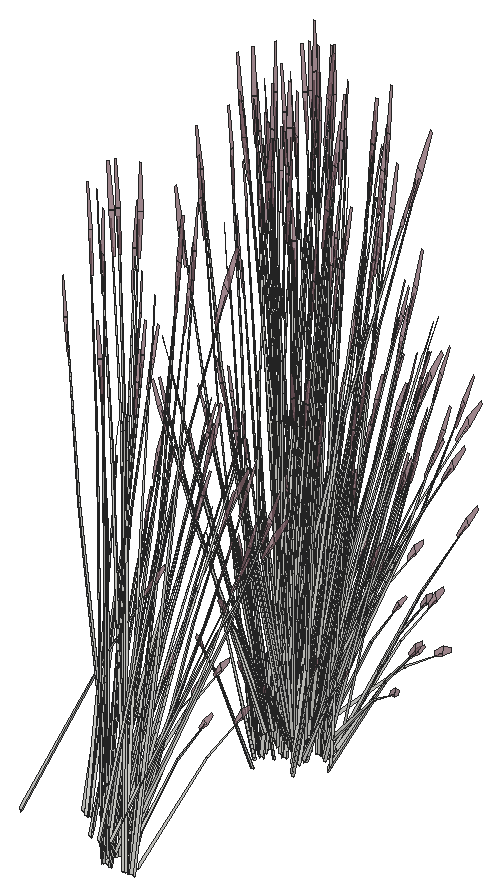
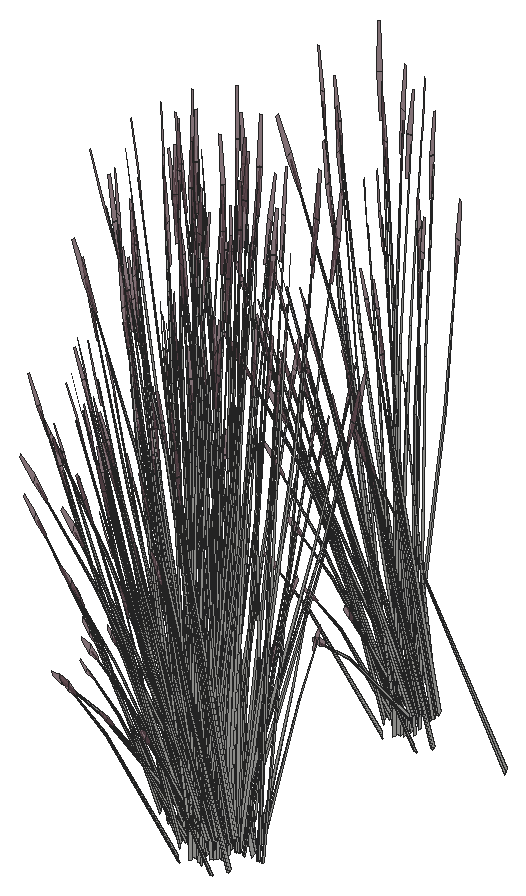
# SketchUp Ruby script. Lengths in inches.
U = 1.inch
M = Sketchup.active_model
def pt(a) = Geom::Point3d.new(a.map { |v| v * U })
def face(e, loops, mat)
  f = e.add_face(loops[0].map { |a| pt(a) })
  loops[1..].each { |l| e.add_face(l.map { |a| pt(a) }).erase! }
  f.material = f.back_material = mat if mat
  f
end
# faces: each face lists its corners as indices into pts; further lists are holes
def faces(e, pts, list, mat = nil) = list.each { |f| face(e, (f[0].is_a?(Array) ? f : [f]).map { |l| l.map { |i| pts[i] } }, mat) }
# xy, xz, yz: faces in a plane at the given z, y or x. An outline is a flat list of corners, or four numbers for a rectangle; further outlines are holes
def ring(l) = l.size == 4 ? [[l[0], l[1]], [l[2], l[1]], [l[2], l[3]], [l[0], l[3]]] : l.each_slice(2).to_a
def flat(e, list, mat, &to3) = list.each { |f| face(e, (f[0].is_a?(Array) ? f : [f]).map { |l| ring(l).map { |u, v| to3.(u, v) } }, mat) }
def xy(e, z, list, mat = nil) = flat(e, list, mat) { |x, y| [x, y, z] }
def xz(e, y, list, mat = nil) = flat(e, list, mat) { |x, z| [x, y, z] }
def yz(e, x, list, mat = nil) = flat(e, list, mat) { |y, z| [x, y, z] }
def lines(e, pts, list) = list.each { |a, b| e.add_line(pt(pts[a]), pt(pts[b])) }
# prism: a flat outline (further loops are holes) pulled along v
def prism(e, loops, v, mat = nil)
  f = face(e, loops, mat); d = Geom::Vector3d.new(v.map { |x| x * U })
  f.pushpull(f.normal.samedirection?(d) ? d.length : -d.length)
end
def box(e, o, s, mat = nil) = prism(e, [[o, [o[0] + s[0], o[1], o[2]], [o[0] + s[0], o[1] + s[1], o[2]], [o[0], o[1] + s[1], o[2]]]], [0, 0, s[2]], mat)
def at(x, y, z, deg = 0) = Geom::Transformation.translation(pt([x, y, z])) * Geom::Transformation.rotation(ORIGIN, Z_AXIS, deg.degrees)
def axes(o, x, y, z) = Geom::Transformation.new([*x, 0, *y, 0, *z, 0, *pt(o).to_a, 1])
def part(name) = M.definitions.add(name)
# library, detail: a bought-in or finely detailed component or shape, given as its bounding box
def library(name, o, s) = part(name).tap { |d| box(d.entities, o, s) }
def detail(e, o, s) = box(e.add_group.entities, o, s)
def put(e, d, t, mat = nil) = e.add_instance(d, t).tap { |i| i.material = mat if mat }
def group(e, t, mat = nil) = e.add_group.tap { |g| g.transformation = t; g.material = mat if mat }.entities
root = M.entities
M.materials.add("LightPink_Translucent").color = [144, 107, 117]
M.materials["LightPink_Translucent"].alpha = 0.75
c1 = part("blade")
p = [[2.15,0.21,22],[0,0.17,0],[0.09,0.45,0],[2.18,0.31,22],[2.29,0.31,22],[0.38,0.45,0],
  [2.48,0.24,33],[2.49,0.24,33],[2.48,0.22,33]]
faces(c1.entities,p,[[0,1,2,3],[4,5,2,3],[6,3,4,7],[8,0,3,6]])
c2 = part("seeds")
p = [[0.3,-0.1,1.38],[-0.01,-0.03,1.59],[-0.01,-0.03,0.03],[0.14,-0.07,-0.07],[0.29,-0.03,3],[0.15,0.01,3.11]]
faces(c2.entities,p,[[0,1,2,3],[1,0,4,5]],"LightPink_Translucent")
c3 = part("blade with seeds")
put(c3.entities,c1,at(0,0,0))
put(c3.entities,c2,axes([2.4,0.25,30.99],[1.5799,-0.05474,1.17369],[-0.12525,1.92788,0.29478],[-0.07173,-0.02425,1.56792]))
put(root,c3,axes([507.35,187.09,1.81],[0.56134,0.36712,0.1448],[-0.46823,0.41419,-0.41347],[-0.13033,0.05599,1.26744]))
put(root,c3,axes([508.8,187.72,4.17],[0.75952,0.01471,-0.71045],[-0.05101,0.61953,0.08574],[0.32177,0.06538,1.00501]))
put(root,c3,axes([507.94,188.22,1.67],[0.7111,-0.30552,0.49651],[0.42504,0.54784,0],[-0.16196,0.06958,1.57504]))
put(root,c3,axes([506.93,187.74,1.48],[0.33034,0.70197,-0.06012],[-0.94388,0.24598,0],[0.01154,0.02451,1.72173]))
put(root,c3,axes([507.3,188.5,1.22],[-0.70886,-0.15119,-0.30978],[0.17848,-0.53243,0.30978],[-0.1429,0.0614,1.38974]))
put(root,c3,axes([510.04,186.47,1.57],[0.95008,0,0],[0,0.68292,-0.51607],[0,0.15554,1.63711]))
put(root,c3,axes([509.66,186.82,1.39],[-0.94962,-0.00489,-0.04976],[0,-0.68292,0.49943],[-0.02984,0.15546,1.58352]))
put(root,c3,axes([507.6,186.22,1.86],[0.85568,0.29155,-0.29095],[-0.41201,0.61537,-0.50002],[0.02689,0.15109,1.59708]))
put(root,c3,axes([509.26,187.98,3.72],[0.43232,0.38257,-0.35414],[-0.49364,0.36215,0.4572],[0.25081,0.0551,0.87481]))
put(root,c3,axes([509.46,186.92,1.22],[-0.53038,0.38124,-0.30978],[-0.53038,-0.38124,0.30978],[0,0.1228,1.38974]))
put(root,c3,axes([507.18,186.95,1.86],[0.08854,0.69723,-0.29095],[-0.92215,0.04216,-0.50002],[-0.16238,0.09287,1.59708]))
put(root,c3,axes([509.03,188.125,3.92],[-0.03826,0.46465,0.0643],[-0.57772,-0.01274,0.50621],[0.2213,0.04862,0.77189]))
put(root,c3,axes([507.51,186.68,1.4],[-0.36864,0.55059,-0.44739],[-0.76598,-0.26498,0.21531],[0,0.12692,1.43643]))
put(root,c3,axes([497.26,188.9,1.78],[-0.18299,-0.15028,1.43002],[0.23809,-0.49714,-0.30754],[0.37023,0.06735,0.61141]))
put(root,c3,axes([509.09,187.98,3.93],[-0.56024,0.40262,0.48003],[-0.48318,-0.42758,0.3958],[0.26285,0.07427,0.9933]))
put(root,c3,axes([507.31,188.44,4.24],[-0.11735,-0.49217,0.35414],[0.67083,-0.12996,-0.4572],[0.18018,0.14104,0.87481]))
put(root,c3,axes([507.53,188.26,1.52],[0.95122,0.19861,0.30756],[-0.23797,0.7099,-0.36492],[-0.15744,0.08885,1.64885]))
put(root,c3,axes([509.83,186.93,1.21],[0,0.61104,-0.49651],[-0.85008,0,0],[0,0.13917,1.57504]))
put(root,c3,axes([507.7,187,3.07],[-0.28223,-0.10528,1.71376],[0.58406,-0.44165,0.13857],[0.36402,0.19924,0.73262]))
put(root,c3,axes([507.76,185.61,3.67],[-0.65655,-0.31748,1.38283],[0.69326,-0.49431,0.59665],[0.21183,0.29789,1.33663]))
put(root,c3,axes([508.75,188.2,1.96],[-0.4278,-0.1757,1.1486],[0.5524,-0.17852,0.84392],[0.14899,0.15122,0.25299]))
put(root,c3,axes([507.24,188.7,4.23],[0.45276,-0.52302,-0.1216],[0.65568,0.30132,-0.67495],[0.22792,0.14777,1.02557]))
put(root,c3,axes([504.26,187.99,4.24],[0.5141,-0.32171,0.35414],[0.48666,0.36734,-0.4572],[-0.07405,0.18664,0.87481]))
put(root,c3,axes([508.11,188.64,1.57],[0.47504,0.61229,0],[-0.79476,0.34146,-0.51607],[-0.18101,0.07777,1.63711]))
put(root,c3,axes([506.65,189.13,3.9],[0.00225,-0.07398,1.77383],[0.65113,-0.32638,-0.16761],[0.22617,0.1165,0.31391]))
put(root,c3,axes([508.87,188.85,0.6875],[0.05536,-0.08822,1.76342],[0.69692,-0.25981,-0.26939],[0.21129,0.13447,0.30037]))
put(root,c3,axes([507.71,186.22,2.03],[-0.02076,-0.57531,1.41272],[0.93937,0.14913,0.59816],[-0.22217,0.31481,1.3335]))
put(root,c3,axes([507.95,186.85,1.29],[0.2786,0.55945,-0.69212],[-0.80253,0.20149,-0.18165],[0.03079,0.18945,1.52773]))
put(root,c3,axes([507.78,188.4375,3.875],[0.74975,-0.14525,-0.51099],[0.13115,0.55007,-0.3958],[0.20138,0.15763,0.97773]))
put(root,c3,axes([505.7,188.52,4.24],[0.22906,-0.4699,0.35414],[0.66828,0.13705,-0.4572],[0.06128,0.18919,0.87481]))
put(root,c3,axes([508.82,189,1.86],[-0.48723,-0.01916,1.0506],[0.32177,-0.40701,0.58006],[0.19248,0.1446,0.8241]))
put(root,c3,axes([507.41,188.89,3.92],[-0.34533,0.38816,0.0643],[-0.49176,-0.22599,0.50621],[0.15898,0.12445,0.77189]))
put(root,c3,axes([506.6,190.2,4.84],[0.52505,-0.35054,-0.06488],[0.48109,0.38392,-0.29416],[0.03387,0.10878,0.97024]))
put(root,c3,axes([507.56,188.78,3.93],[-0.75571,0.14023,0.48003],[-0.13115,-0.55007,0.3958],[0.17773,0.16212,0.9933]))
put(root,c3,axes([507.22,188.01,1.78],[0.01341,-0.20255,1.43002],[0.64074,-0.22625,-0.30754],[0.1978,0.24243,0.61141]))
put(root,c3,axes([505.49,188.95,3.92],[-0.55987,0.20767,0.0643],[-0.27403,-0.37869,0.50621],[0.05407,0.16693,0.77189]))
put(root,c3,axes([503.93,188.08,4.59],[0.83505,0.03027,-0.13498],[-0.02282,0.57322,-0.74919],[-0.05801,0.22077,1.13838]))
put(root,c3,axes([505.48,188.72,4.23],[0.74352,-0.28449,-0.1216],[0.36538,0.50492,-0.67495],[0.0981,0.21277,1.02557]))
put(root,c3,axes([505.69,188.91,4.26],[-0.74868,-0.15974,0.53283],[0.25601,-0.52518,0.43934],[0.04499,0.20653,1.10256]))
put(root,c3,axes([505.61,188.83,0.6875],[0.12297,-0.03325,1.76342],[0.73967,0.18301,-0.26939],[0.02163,0.20626,0.30037]))
put(root,c3,axes([504.5,188.3,4.2],[0.54391,0.41056,-0.5672],[-0.57458,0.35956,-0.43934],[-0.08276,0.2086,1.08528]))
put(root,c3,axes([503.91,188.91,2.02],[0.69024,-0.1082,0.06507],[0.15868,0.43593,-0.86304],[-0.04376,0.22067,0.7736]))
put(root,c3,axes([506.12,188.69,3.875],[0.7469,0.15318,-0.51099],[-0.25601,0.52518,-0.3958],[0.06849,0.21144,0.97773]))
put(root,c3,axes([506.54,187.61,3.07],[-0.17368,-0.19618,1.71376],[0.80256,-0.16516,0.13857],[0.18139,0.30799,0.73262]))
put(root,c3,axes([505.78,189.02,3.72],[-0.22906,0.4699,-0.35414],[-0.66828,-0.13705,0.4572],[0.06128,0.18919,0.87481]))
put(root,c3,axes([505.12,187.71,3.07],[-0.0186,-0.23452,1.71376],[0.80601,0.15558,0.13857],[-0.04985,0.33422,0.73262]))
put(root,c3,axes([505.84,188.59,4.17],[0.36264,0.49684,-0.71045],[-0.74649,0.27689,0.08574],[0.0848,0.24006,1.00501]))
put(root,c3,axes([505.3,189.85,3.91],[0.09631,0.0984,1.74944],[0.77725,0.03866,-0.27667],[0.07816,0.217,0.14031]))
put(root,c3,axes([507.89,207.74,1.78],[-0.21597,0.12368,1.43002],[-0.64681,-0.21647,-0.30754],[0.1199,-0.26922,0.61141]))
put(root,c3,axes([506.9,208.17,4.17],[-0.36264,-0.49684,-0.71045],[0.74649,-0.27689,0.08574],[-0.0848,-0.24006,1.00501]))
put(root,c3,axes([506.28,207.06,0.6875],[-0.12744,0.02202,1.76342],[-0.70477,-0.24781,-0.26939],[0.01183,-0.2067,0.30037]))
put(root,c3,axes([508.41,208.65,4.17],[0.01977,-0.56521,-0.71045],[0.83252,0.03796,0.08574],[0.08786,-0.23945,1.00501]))
put(root,c3,axes([509.57,207.77,3.91],[-0.00733,-0.12161,1.74944],[-0.61946,-0.35147,-0.27667],[0.09577,-0.21306,0.14031]))
put(root,c3,axes([506.97,207.74,3.72],[0.22906,-0.4699,-0.35414],[0.66828,0.13705,0.4572],[-0.06128,-0.18919,0.87481]))
put(root,c3,axes([507.47,208.37,3.07],[-0.14147,0.21002,1.71376],[-0.59349,-0.43464,0.13857],[0.26773,-0.27089,0.73262]))
put(root,c3,axes([509.41,207.33,3.9],[-0.07716,0.04667,1.77383],[-0.75601,-0.15746,-0.16761],[-0.02737,-0.20368,0.31391]))
put(root,c3,axes([506.63,208.07,3.875],[-0.7469,-0.15318,-0.51099],[0.25601,-0.52518,-0.3958],[-0.06849,-0.21144,0.97773]))
put(root,c3,axes([507.09,206.75,1.96],[0.09747,0.35631,1.1486],[-0.54071,-0.19735,0.84392],[0.05818,-0.18244,0.25299]))
put(root,c3,axes([508.24,208.46,3.875],[-0.54391,-0.41056,-0.51099],[0.57458,-0.35956,-0.3958],[0.08276,-0.2086,0.97773]))
put(root,c3,axes([507.05,207.85,3.93],[0.74868,0.15974,0.48003],[-0.25601,0.52518,0.3958],[-0.04499,-0.20653,0.9933]))
put(root,c3,axes([507.27,208.04,4.23],[-0.74352,0.28449,-0.1216],[-0.36538,-0.50492,-0.67495],[-0.0981,-0.21277,1.02557]))
put(root,c3,axes([508.8125,208.68,4.23],[-0.83505,-0.03027,-0.1216],[0.02282,-0.57322,-0.67495],[0.05801,-0.22077,1.02557]))
put(root,c3,axes([508.75,208.3125,3.72],[0.5141,-0.32171,-0.35414],[0.48666,0.36734,0.4572],[0.07405,-0.18664,0.87481]))
put(root,c3,axes([507.25,207.8125,3.92],[0.55987,-0.20767,0.0643],[0.27403,0.37869,0.50621],[-0.05407,-0.16693,0.77189]))
put(root,c3,axes([505.22,210.03,1.29],[-0.31203,-0.62659,-0.69835],[0.89884,-0.22566,-0.18329],[-0.03449,-0.21218,1.54149]))
put(root,c3,axes([509.4,208.12,0.6875],[-0.11372,-0.04814,1.76342],[-0.29211,-0.53779,-0.26939],[0.19706,-0.14594,0.30037]))
put(root,c3,axes([507.04,208.24,4.24],[-0.22906,0.4699,0.35414],[-0.66828,-0.13705,-0.4572],[-0.06128,-0.18919,0.87481]))
put(root,c3,axes([508.75,208.4375,3.93],[0.54105,0.41691,0.48003],[-0.57458,0.35956,0.3958],[0.0998,-0.1956,0.9933]))
put(root,c3,axes([508.95,208.48,3.92],[0.62439,0.02847,0.0643],[-0.01712,0.42991,0.50621],[0.06534,-0.16468,0.77189]))
put(root,c3,axes([508.49,208.77,4.24],[-0.5141,0.32171,0.35414],[-0.48666,-0.36734,-0.4572],[0.07405,-0.18664,0.87481]))
put(root,c3,axes([509.39,209.64,4.17],[0.39688,-0.48213,-0.71045],[0.69548,0.34264,0.08574],[0.23697,-0.17468,1.00501]))
put(root,c3,axes([505.1,208.23,1.57],[-0.47504,-0.61229,0],[0.79476,-0.34146,-0.51607],[0.18101,-0.07777,1.63711]))
put(root,c3,axes([509.37,209.41,3.875],[-0.19519,-0.55794,-0.51099],[0.73919,-0.0976,-0.3958],[0.21183,-0.14986,0.97773]))
put(root,c3,axes([506.14,207.49,1.32],[-0.52505,0.35054,-0.03893],[-0.48109,-0.38392,-0.17649],[-0.03387,-0.10878,0.58215]))
put(root,c3,axes([509.72,209.81,4.23],[-0.70283,-0.33692,-0.1216],[0.40491,-0.48793,-0.67495],[0.19857,-0.16961,1.02557]))
put(root,c3,axes([503.38,209.95,1.21],[0,-0.61104,-0.49651],[0.85008,0,0],[0,-0.13917,1.57504]))
put(root,c3,axes([505.75,208.14,1.21],[0.7111,-0.30552,-0.49651],[0.42504,0.54784,0],[0.16196,-0.06958,1.57504]))
put(root,c3,axes([509.97,209.19,1.78],[-0.27143,-0.0181,1.43002],[-0.27808,-0.48551,-0.30754],[0.33346,-0.13735,0.61141]))
put(root,c3,axes([511.45,209.66,3.9],[-0.09924,-0.00464,1.77383],[-0.4121,-0.49725,-0.16761],[0.1655,-0.1635,0.31391]))
put(root,c3,axes([506.59,209.39,1.25],[0.51177,-0.45928,-0.62353],[0.63575,0.41646,-0.16365],[0.20507,-0.11457,1.37633]))
put(root,c3,axes([510.28,208.3,1.96],[-0.25308,0.31105,1.1486],[-0.21753,-0.4179,0.84392],[0.20902,-0.10472,0.25299]))
put(root,c3,axes([509.92,209.47,3.72],[0.66138,-0.08733,-0.35414],[0.17464,0.49921,0.4572],[0.18953,-0.13408,0.87481]))
put(root,c3,axes([505.7,210.19,1.4],[0.36864,-0.55059,-0.44739],[0.76598,0.26498,0.21531],[0,-0.12692,1.43643]))
put(root,c3,axes([506.04,209.92,1.86],[-0.08854,-0.69723,-0.29095],[0.92215,-0.04216,-0.50002],[0.16238,-0.09287,1.59708]))
put(root,c3,axes([503.75,209.96,1.22],[0.53038,-0.38124,-0.30978],[0.53038,0.38124,0.30978],[0,-0.1228,1.38974]))
put(root,c3,axes([509.38,209.76,4.24],[-0.66138,0.08733,0.35414],[-0.17464,-0.49921,-0.4572],[0.18953,-0.13408,0.87481]))
put(root,c3,axes([505.61,210.65,1.86],[-0.85568,-0.29155,-0.29095],[0.41201,-0.61537,-0.50002],[-0.02689,-0.15109,1.59708]))
put(root,c3,axes([505.91,208.38,1.22],[0.70886,0.15119,-0.30978],[-0.17848,0.53243,0.30978],[0.1429,-0.0614,1.38974]))
put(root,c3,axes([509.98,209.68,3.92],[0.52161,0.25698,0.0643],[-0.30368,0.36595,0.50621],[0.16723,-0.11831,0.77189]))
put(root,c3,axes([509.83,209.58,3.93],[0.18844,0.56237,0.48003],[-0.73919,0.0976,0.3958],[0.21785,-0.13226,0.9933]))
put(root,c3,axes([511.83,210.26,3.91],[0.10543,-0.09307,1.74944],[-0.13495,-0.57092,-0.27667],[0.26455,-0.10825,0.14031]))
put(root,c3,axes([506.16,210.47,1.625],[0.8561,0.29616,0.24065],[-0.41201,0.61537,0.50002],[0,-0.14185,1.60543]))
put(root,c3,axes([505.88,210.06,1.91],[-0.82508,0.03772,0.44739],[-0.07462,-0.62614,-0.21531],[0.14771,-0.06346,1.43643]))
put(root,c3,axes([503.75,210.51,1.67],[0,0.61104,0.49651],[-0.85008,0,0],[0,-0.13917,1.57504]))
put(root,c3,axes([509.75,211.125,4.23],[-0.38229,-0.5533,-0.1216],[0.6785,-0.2719,-0.67495],[0.28593,-0.073,1.02557]))
put(root,c3,axes([509.72,210.65,3.875],[0.20584,-0.55581,-0.51099],[0.70573,0.19051,-0.3958],[0.28414,-0.05097,0.97773]))
put(root,c3,axes([508.6,208.39,1.57],[0.47504,-0.61229,0],[0.79476,0.34146,-0.51607],[0.18101,0.07777,1.63711]))
put(root,c3,axes([505.85,210.28,1.55],[0.33034,0.68327,0.45755],[-0.94388,0.2376,0.17955],[0.01154,-0.12555,1.58856]))
put(root,c3,axes([510.47,210.81,1.17],[-0.48937,0.07333,1.41583],[-0.07789,-0.58369,0.08104],[0.34275,-0.08835,0.80566]))
put(root,c3,axes([511.36,210.29,1.45],[-0.47106,-0.39072,-0.06488],[0.51591,-0.35801,-0.29416],[0.14618,-0.02521,0.97024]))
put(root,c3,axes([505.68,210.82,1.91],[-0.36864,0.55059,0.44739],[-0.76598,-0.26498,-0.21531],[0,-0.12692,1.43643]))
put(root,c3,axes([507.04,210.34,1.4],[0,-0.70701,0],[0.95008,0,0],[0,0,1.79456]))
put(root,c3,axes([508.19,208.71,1.67],[-0.7111,-0.30552,0.49651],[0.42504,-0.54784,0],[0.16196,0.06958,1.57504]))
put(root,c3,axes([509.58,210.85,4.17],[0.66765,-0.26986,-0.71045],[0.37208,0.55551,0.08574],[0.32259,-0.0631,1.00501]))
put(root,c3,axes([506.59,209.89,1.55],[-0.62999,0.55453,0.45755],[-0.74845,-0.4895,0.17955],[0.15188,-0.05534,1.58856]))
put(root,c3,axes([507.28,210.89,1.49],[-0.70674,-0.52593,-0.06131],[0.70717,-0.52625,0],[-0.02468,-0.01837,1.75571]))
put(root,c3,axes([505.49,208.98,1.67],[-0.21949,0.60727,0.17642],[-0.8032,-0.17185,0.35086],[0.13875,-0.00296,1.60407]))
put(root,c3,axes([509.48,210.96,4.24],[-0.63144,-0.17046,0.35414],[0.18417,-0.49731,-0.4572],[0.25423,-0.0456,0.87481]))
put(root,c3,axes([505.16,209.47,0.79],[-0.74787,0.24464,1.28929],[-0.23804,-0.70192,0.50096],[0.45924,0.01168,1.46642]))
put(root,c3,axes([507.17,209.66,1.81],[0.14658,-0.54532,0.1448],[0.71613,0.09466,-0.41347],[0.13033,0.05599,1.26744]))
put(root,c3,axes([505.93,210.95,1.55],[0.96033,0.12874,0.45755],[-0.19544,0.7271,0.17955],[-0.14034,-0.07021,1.58856]))
put(root,c3,axes([511,210.42,0.6875],[-0.03971,-0.09277,1.76342],[0.27541,-0.54264,-0.26939],[0.27782,-0.00781,0.30037]))
put(root,c3,axes([506.87,209.8,1.91],[-0.45644,-0.51287,0.44739],[0.69137,-0.36116,-0.21531],[0.14771,0.06346,1.43643]))
put(root,c3,axes([505.42,212.11,1.67],[0.81646,-0.16218,0.17642],[0.20161,0.60355,0.35086],[-0.07282,-0.08794,1.60407]))
put(root,c3,axes([507.1,209.83,1.86],[0.76714,-0.40567,-0.29095],[0.51013,0.57321,-0.50002],[0.18927,0.05821,1.59708]))
put(root,c3,axes([510.15,210.9,3.72],[0.63144,0.17046,-0.35414],[-0.18417,0.49731,0.4572],[0.25423,-0.0456,0.87481]))
put(root,c3,axes([509.03,208.75,1.21],[0.7111,0.30552,-0.49651],[-0.42504,0.54784,0],[0.16196,0.06958,1.57504]))
put(root,c3,axes([507.68,210.5,1.4],[0.85008,0,0],[0,0.63259,0],[0,0,1.78407]))
put(root,c3,axes([507.92,209.01,1.67],[-0.81646,0.16218,0.17642],[-0.20161,-0.60355,0.35086],[0.07282,0.08794,1.60407]))
put(root,c3,axes([508.43,210.29,3.07],[-0.31515,0.01384,1.71376],[0.20907,-0.5998,0.13857],[0.44912,0.0371,0.73262]))
put(root,c3,axes([508.83,208.98,1.22],[0.17848,0.53243,-0.30978],[-0.70886,0.15119,0.30978],[0.1429,0.0614,1.38974]))
put(root,c3,axes([510.06,211.11,3.92],[0.27906,0.41663,0.0643],[-0.50888,0.20393,0.50621],[0.22432,-0.04024,0.77189]))
put(root,c3,axes([507.41,210.18,1.57],[-0.96033,-0.12874,0.49198],[0.19544,-0.7271,0.19306],[0.14034,0.07021,1.70813]))
put(root,c3,axes([510,210.96,3.93],[-0.21466,0.55714,0.48003],[-0.70573,-0.19051,0.3958],[0.27753,-0.03348,0.9933]))
put(root,c3,axes([506.64,211.97,1.4],[-0.24791,-0.5268,0],[0.70791,-0.18448,0],[0,0,1.54371]))
put(root,c3,axes([507.57,211.9,1.38],[0.79769,-0.20732,-0.19198],[0.2803,0.59721,0.00008],[0.08805,-0.02292,1.73897]))
put(root,c3,axes([507.85,212.15,1.67],[0.21949,-0.60727,0.17642],[0.8032,0.17185,0.35086],[-0.13875,0.00296,1.60407]))
put(root,c3,axes([507.66,210.77,1.41],[0.53038,0.39469,0],[-0.53038,0.39469,0],[0,0,1.69266]))
put(root,c3,axes([509.1,210.6,1.67],[-0.59697,-0.44509,0.17642],[0.60159,-0.4317,0.35086],[-0.06593,0.0909,1.60407]))
put(root,c3,axes([508,209.92,1.25],[0.79037,0.10018,-0.62353],[-0.16679,0.61794,-0.16365],[0.23587,0.07488,1.37633]))
put(root,c3,axes([511.49,211,1.96],[-0.46945,0.10088,1.1486],[0.22097,-0.4169,0.84392],[0.24904,0.02853,0.25299]))
put(root,c3,axes([506.47,212.21,1.39],[-0.76598,-0.27433,0],[0.36864,-0.57001,0],[0,0,1.62707]))
put(root,c3,axes([507.66,210.31,1.91],[0.36864,-0.55059,0.44739],[0.76598,0.26498,-0.21531],[0,0.12692,1.43643]))
put(root,c3,axes([511.27,212.77,3.9],[-0.0687,-0.05349,1.77383],[0.15029,-0.57341,-0.16761],[0.27062,-0.03664,0.31391]))
put(root,c3,axes([507.52,210.62,1.48],[0,0.70667,-0.05637],[-0.95008,0,0],[0,0.02221,1.79368]))
put(root,c3,axes([507.59,210.12,1.4],[0.45644,0.51287,-0.44739],[-0.69137,0.36116,0.21531],[0.14771,0.06346,1.43643]))
put(root,c3,axes([510.67,212.29,3.12],[-0.14542,-0.51365,-0.03492],[0.68734,-0.11809,-0.15832],[0.14353,0.03256,0.52218]))
put(root,c3,axes([508.89,212.27,4.23],[0.04068,-0.62141,-0.1216],[0.77029,0.01698,-0.67495],[0.29667,0.04317,1.02557]))
put(root,c3,axes([509.59,210.61,1.67],[0,-0.61104,0.49651],[0.85008,0,0],[0,0.13917,1.57504]))
put(root,c3,axes([507.46,211.07,1.91],[0.82508,-0.03772,0.44739],[0.07462,0.62614,-0.21531],[-0.14771,0.06346,1.43643]))
put(root,c3,axes([507.98,210.43,1.81],[0.70791,-0.1782,0.1448],[0.24791,0.50885,-0.41347],[0,0.11199,1.26744]))
put(root,c3,axes([508.77,212.03,4.24],[-0.43232,-0.38257,0.35414],[0.49364,-0.36215,-0.4572],[0.25081,0.0551,0.87481]))
put(root,c3,axes([510.61,211.67,1.78],[-0.18299,-0.15028,1.43002],[0.23809,-0.49714,-0.30754],[0.37023,0.06735,0.61141]))
put(root,c3,axes([507.34,212.22,1.4],[0.76598,0.27433,0],[-0.36864,0.57001,0],[0,0,1.74954]))
put(root,c3,axes([509.5625,211.9,3.91],[0.16299,-0.01033,1.74944],[0.44707,-0.47471,-0.27667],[0.28992,0.06266,0.14031]))
put(root,c3,axes([507.64,212.83,1.39],[-0.46912,-0.61443,-0.05142],[0.79476,-0.34146,0.51607],[-0.19584,0.0585,1.6363]))
put(root,c3,axes([507.48,211.34,1.81],[0.56134,0.36712,0.1448],[-0.46823,0.41419,-0.41347],[-0.13033,0.05599,1.26744]))
put(root,c3,axes([508.93,211.97,4.17],[0.75952,0.01471,-0.71045],[-0.05101,0.61953,0.08574],[0.32177,0.06538,1.00501]))
put(root,c3,axes([508.07,212.47,1.67],[0.7111,-0.30552,0.49651],[0.42504,0.54784,0],[-0.16196,0.06958,1.57504]))
put(root,c3,axes([507.0625,211.99,1.48],[0.33034,0.70197,-0.06012],[-0.94388,0.24598,0],[0.01154,0.02451,1.72173]))
put(root,c3,axes([507.43,212.75,1.22],[-0.70886,-0.15119,-0.30978],[0.17848,-0.53243,0.30978],[-0.1429,0.0614,1.38974]))
put(root,c3,axes([510.17,210.72,1.57],[0.95008,0,0],[0,0.68292,-0.51607],[0,0.15554,1.63711]))
put(root,c3,axes([509.79,211.07,1.39],[-0.94962,-0.00489,-0.04976],[0,-0.68292,0.49943],[-0.02984,0.15546,1.58352]))
put(root,c3,axes([507.74,210.47,1.86],[0.85568,0.29155,-0.29095],[-0.41201,0.61537,-0.50002],[0.02689,0.15109,1.59708]))
put(root,c3,axes([509.39,212.23,3.72],[0.43232,0.38257,-0.35414],[-0.49364,0.36215,0.4572],[0.25081,0.0551,0.87481]))
put(root,c3,axes([509.59,211.17,1.22],[-0.53038,0.38124,-0.30978],[-0.53038,-0.38124,0.30978],[0,0.1228,1.38974]))
put(root,c3,axes([507.31,211.2,1.86],[0.08854,0.69723,-0.29095],[-0.92215,0.04216,-0.50002],[-0.16238,0.09287,1.59708]))
put(root,c3,axes([509.16,212.375,3.92],[-0.03826,0.46465,0.0643],[-0.57772,-0.01274,0.50621],[0.2213,0.04862,0.77189]))
put(root,c3,axes([507.64,210.93,1.4],[-0.36864,0.55059,-0.44739],[-0.76598,-0.26498,0.21531],[0,0.12692,1.43643]))
put(root,c3,axes([509.22,212.23,3.93],[-0.56024,0.40262,0.48003],[-0.48318,-0.42758,0.3958],[0.26285,0.07427,0.9933]))
put(root,c3,axes([507.4375,212.69,4.24],[-0.11735,-0.49217,0.35414],[0.67083,-0.12996,-0.4572],[0.18018,0.14104,0.87481]))
put(root,c3,axes([507.66,212.51,1.52],[0.95122,0.19861,0.30756],[-0.23797,0.7099,-0.36492],[-0.15744,0.08885,1.64885]))
put(root,c3,axes([507.6,212.99,1.21],[-0.7111,0.30552,-0.49651],[-0.42504,-0.54784,0],[-0.16196,0.06958,1.57504]))
put(root,c3,axes([509.96,211.18,1.21],[0,0.61104,-0.49651],[-0.85008,0,0],[0,0.13917,1.57504]))
put(root,c3,axes([507.83,211.25,3.07],[-0.28223,-0.10528,1.71376],[0.58406,-0.44165,0.13857],[0.36402,0.19924,0.73262]))
put(root,c3,axes([507.89,209.86,3.67],[-0.65655,-0.31748,1.38283],[0.69326,-0.49431,0.59665],[0.21183,0.29789,1.33663]))
put(root,c3,axes([508.88,212.45,1.96],[-0.4278,-0.1757,1.1486],[0.5524,-0.17852,0.84392],[0.14899,0.15122,0.25299]))
put(root,c3,axes([507.375,212.95,4.23],[0.45276,-0.52302,-0.1216],[0.65568,0.30132,-0.67495],[0.22792,0.14777,1.02557]))
put(root,c3,axes([504.39,212.24,4.24],[0.5141,-0.32171,0.35414],[0.48666,0.36734,-0.4572],[-0.07405,0.18664,0.87481]))
put(root,c3,axes([508.24,212.9,1.57],[0.47504,0.61229,0],[-0.79476,0.34146,-0.51607],[-0.18101,0.07777,1.63711]))
put(root,c3,axes([506.78,213.38,3.9],[0.00225,-0.07398,1.77383],[0.65113,-0.32638,-0.16761],[0.22617,0.1165,0.31391]))
put(root,c3,axes([509,213.1,0.6875],[0.05536,-0.08822,1.76342],[0.69692,-0.25981,-0.26939],[0.21129,0.13447,0.30037]))
put(root,c3,axes([507.84,210.47,2.03],[-0.02076,-0.57531,1.41272],[0.93937,0.14913,0.59816],[-0.22217,0.31481,1.3335]))
put(root,c3,axes([508.08,211.1,1.29],[0.2786,0.55945,-0.69212],[-0.80253,0.20149,-0.18165],[0.03079,0.18945,1.52773]))
put(root,c3,axes([507.91,212.69,3.875],[0.74975,-0.14525,-0.51099],[0.13115,0.55007,-0.3958],[0.20138,0.15763,0.97773]))
put(root,c3,axes([505.83,212.77,4.24],[0.22906,-0.4699,0.35414],[0.66828,0.13705,-0.4572],[0.06128,0.18919,0.87481]))
put(root,c3,axes([508.95,213.25,1.86],[-0.48723,-0.01916,1.0506],[0.32177,-0.40701,0.58006],[0.19248,0.1446,0.8241]))
put(root,c3,axes([507.54,213.14,3.92],[-0.34533,0.38816,0.0643],[-0.49176,-0.22599,0.50621],[0.15898,0.12445,0.77189]))
put(root,c3,axes([506.73,214.45,4.84],[0.52505,-0.35054,-0.06488],[0.48109,0.38392,-0.29416],[0.03387,0.10878,0.97024]))
put(root,c3,axes([507.6875,213.03,3.93],[-0.75571,0.14023,0.48003],[-0.13115,-0.55007,0.3958],[0.17773,0.16212,0.9933]))
put(root,c3,axes([507.35,212.26,1.78],[0.01341,-0.20255,1.43002],[0.64074,-0.22625,-0.30754],[0.1978,0.24243,0.61141]))
put(root,c3,axes([505.625,213.2,3.92],[-0.55987,0.20767,0.0643],[-0.27403,-0.37869,0.50621],[0.05407,0.16693,0.77189]))
put(root,c3,axes([504.0625,212.33,4.59],[0.83505,0.03027,-0.13498],[-0.02282,0.57322,-0.74919],[-0.05801,0.22077,1.13838]))
put(root,c3,axes([505.61,212.97,4.23],[0.74352,-0.28449,-0.1216],[0.36538,0.50492,-0.67495],[0.0981,0.21277,1.02557]))
put(root,c3,axes([505.82,213.16,4.26],[-0.74868,-0.15974,0.53283],[0.25601,-0.52518,0.43934],[0.04499,0.20653,1.10256]))
put(root,c3,axes([505.74,213.08,0.6875],[0.12297,-0.03325,1.76342],[0.73967,0.18301,-0.26939],[0.02163,0.20626,0.30037]))
put(root,c3,axes([504.63,212.55,4.2],[0.54391,0.41056,-0.5672],[-0.57458,0.35956,-0.43934],[-0.08276,0.2086,1.08528]))
put(root,c3,axes([504.04,213.16,2.02],[0.69024,-0.1082,0.06507],[0.15868,0.43593,-0.86304],[-0.04376,0.22067,0.7736]))
put(root,c3,axes([506.25,212.95,3.875],[0.7469,0.15318,-0.51099],[-0.25601,0.52518,-0.3958],[0.06849,0.21144,0.97773]))
put(root,c3,axes([506.67,211.86,3.07],[-0.17368,-0.19618,1.71376],[0.80256,-0.16516,0.13857],[0.18139,0.30799,0.73262]))
put(root,c3,axes([505.91,213.27,3.72],[-0.22906,0.4699,-0.35414],[-0.66828,-0.13705,0.4572],[0.06128,0.18919,0.87481]))
put(root,c3,axes([505.25,211.96,3.07],[-0.0186,-0.23452,1.71376],[0.80601,0.15558,0.13857],[-0.04985,0.33422,0.73262]))
